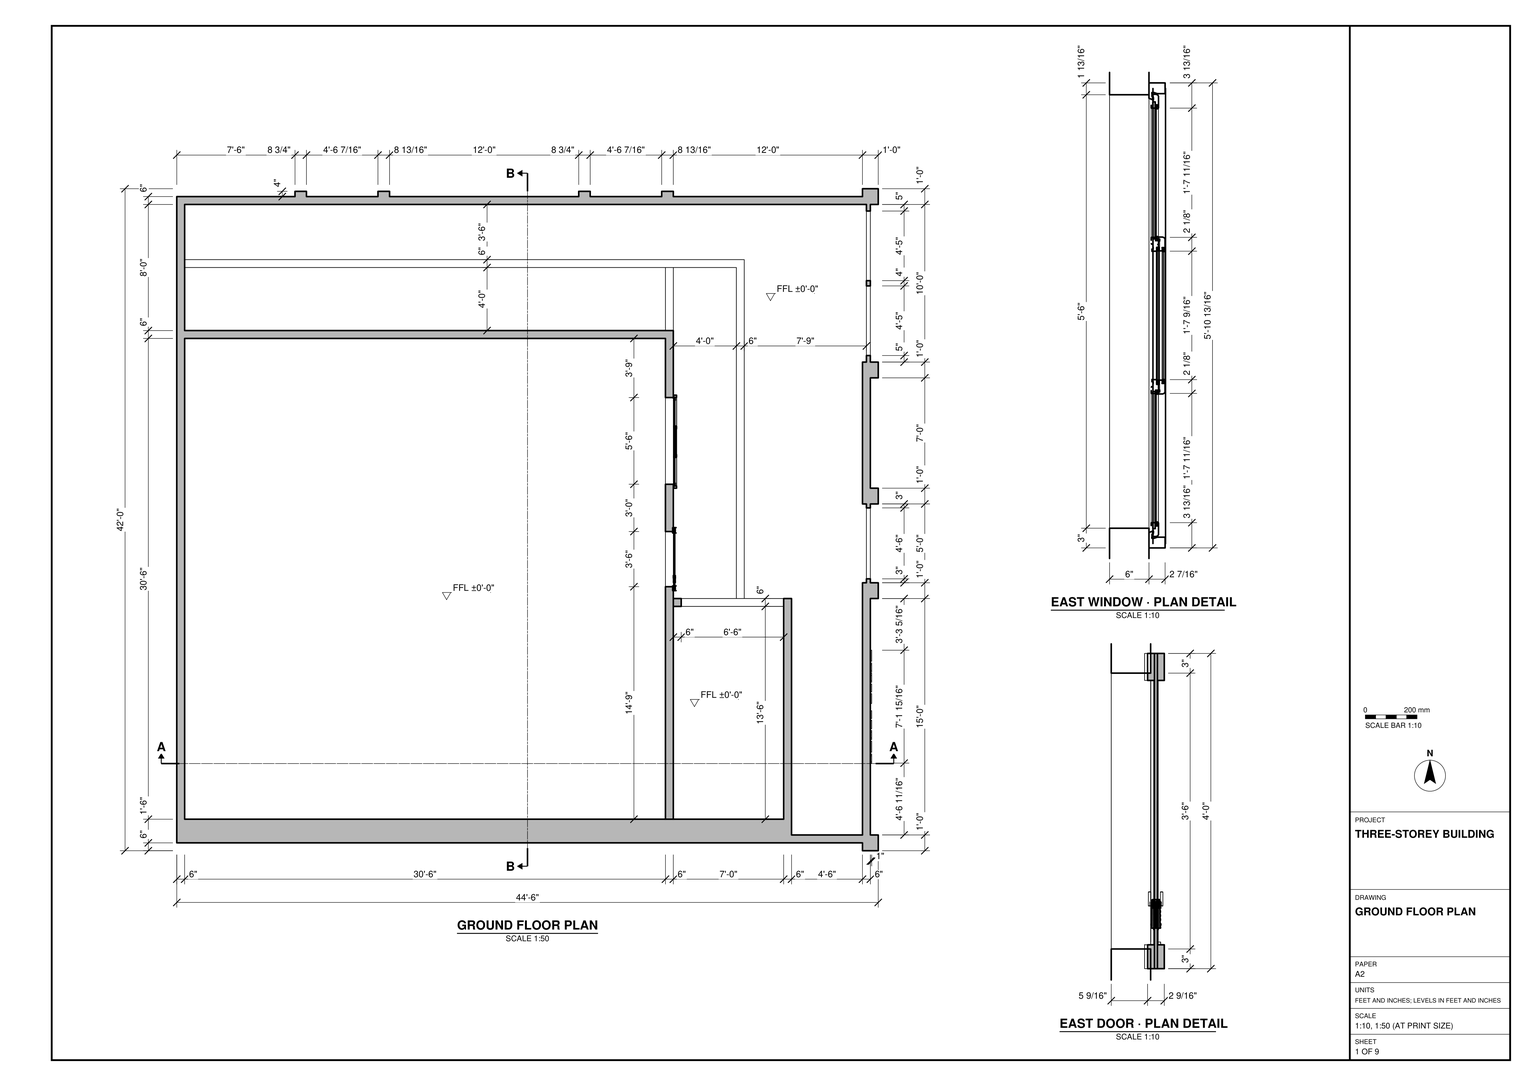
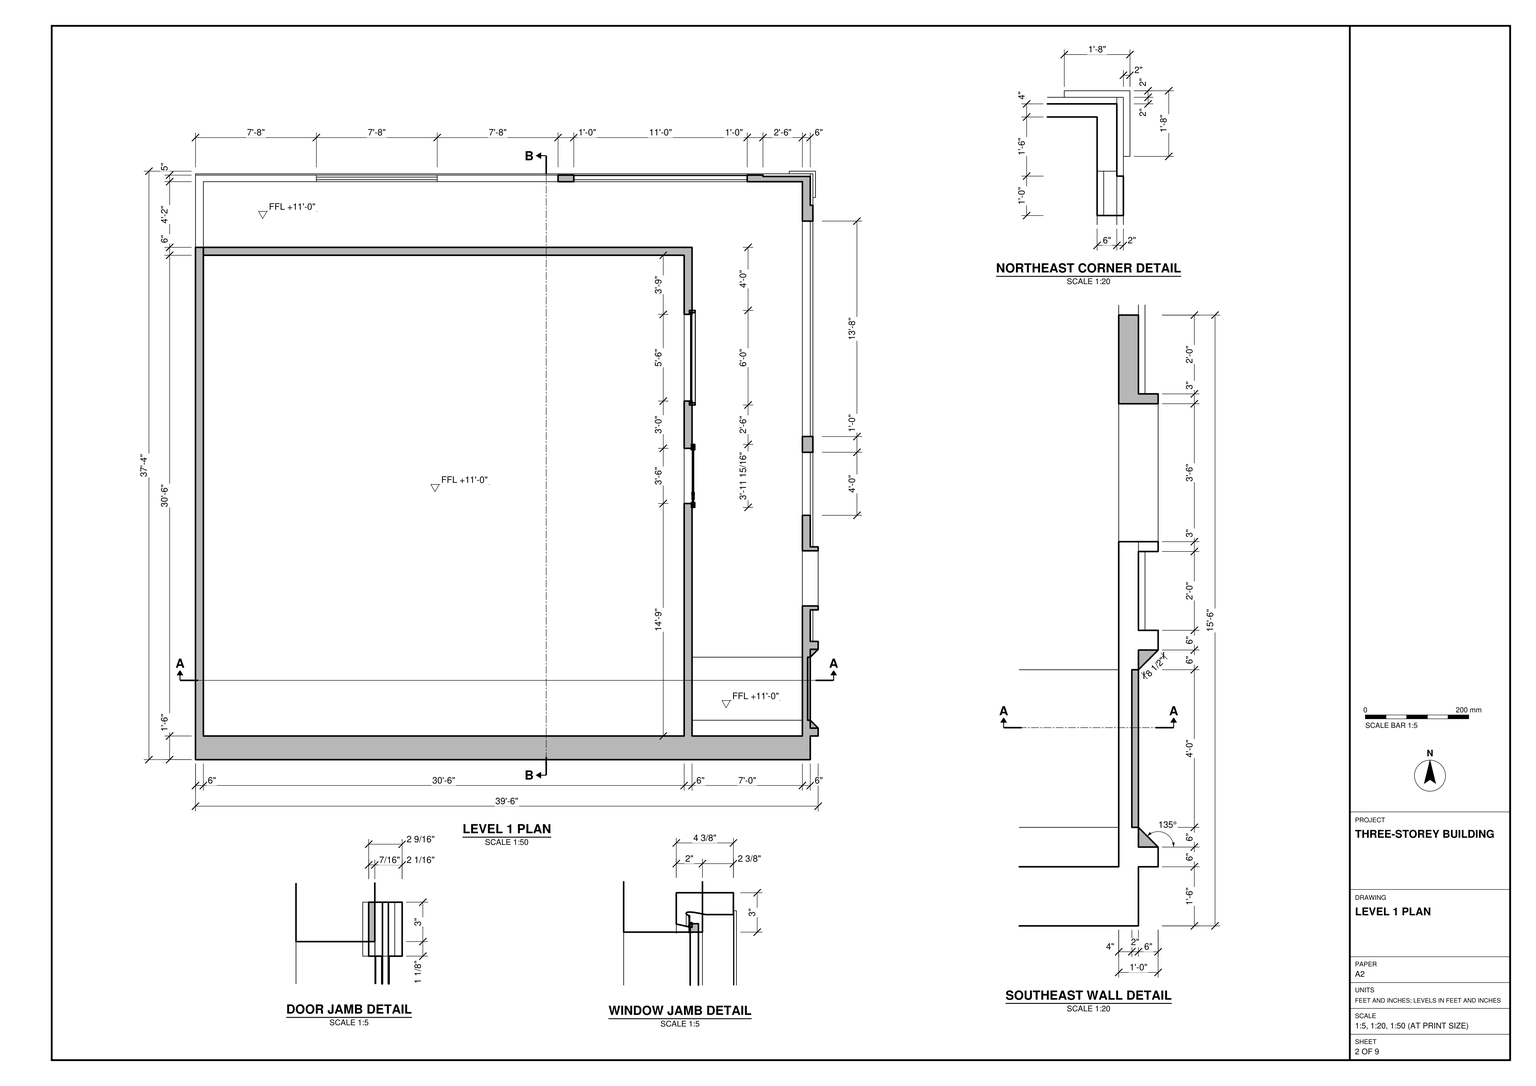
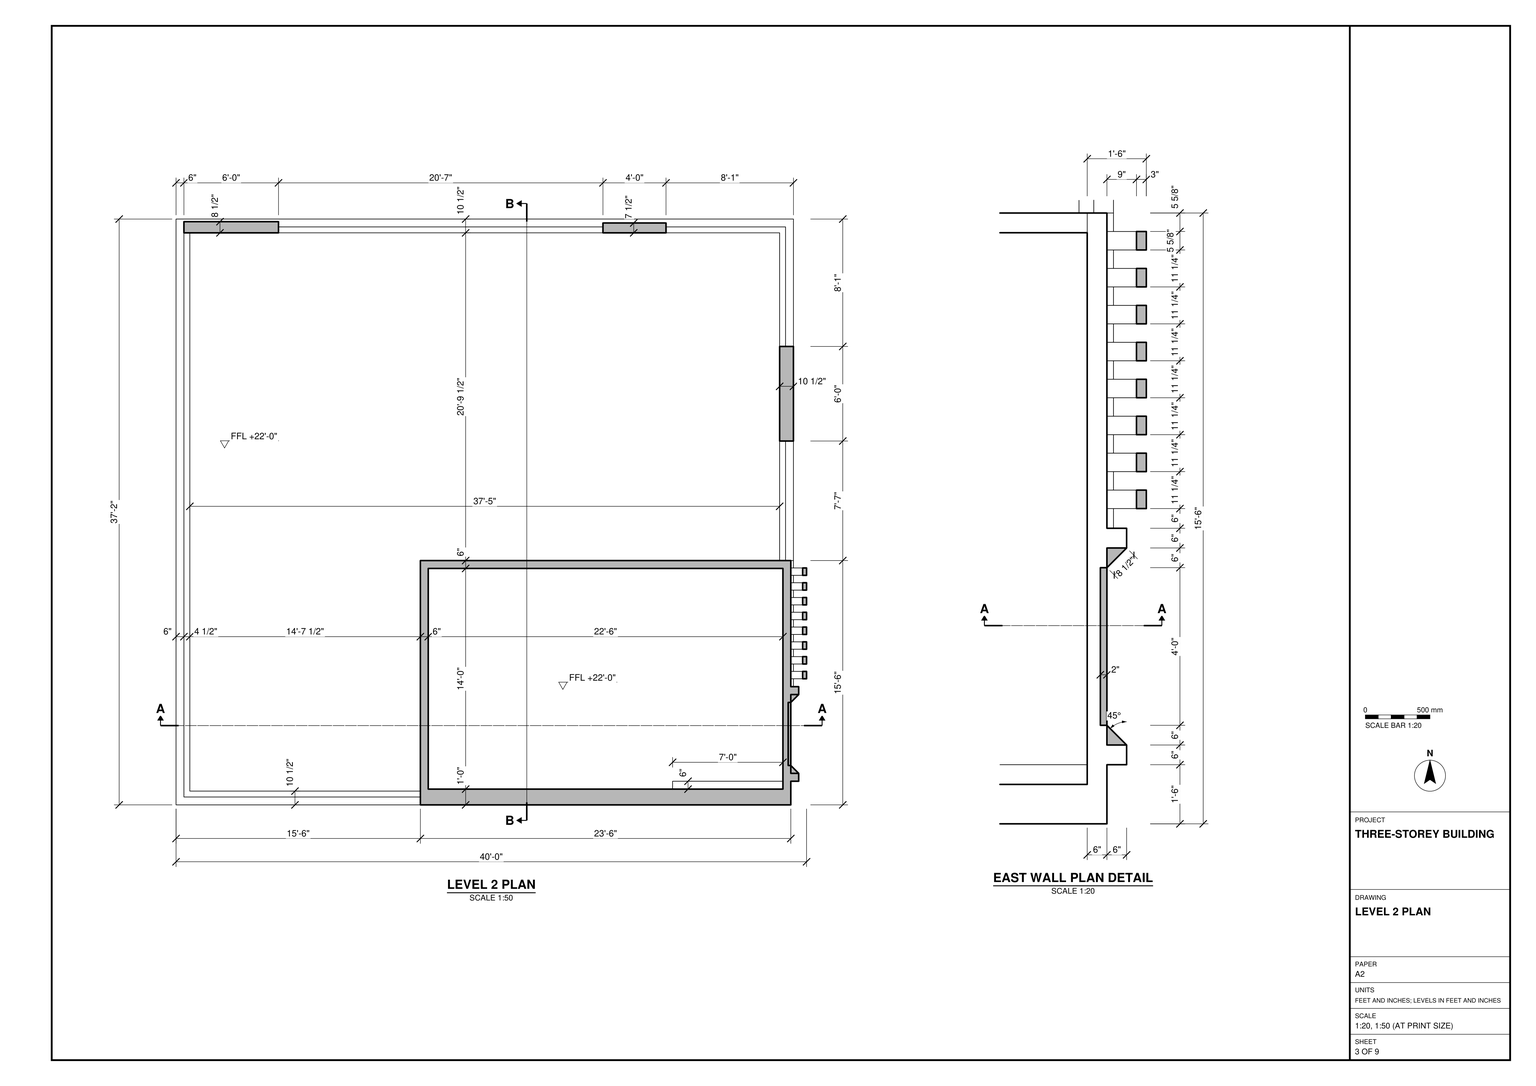
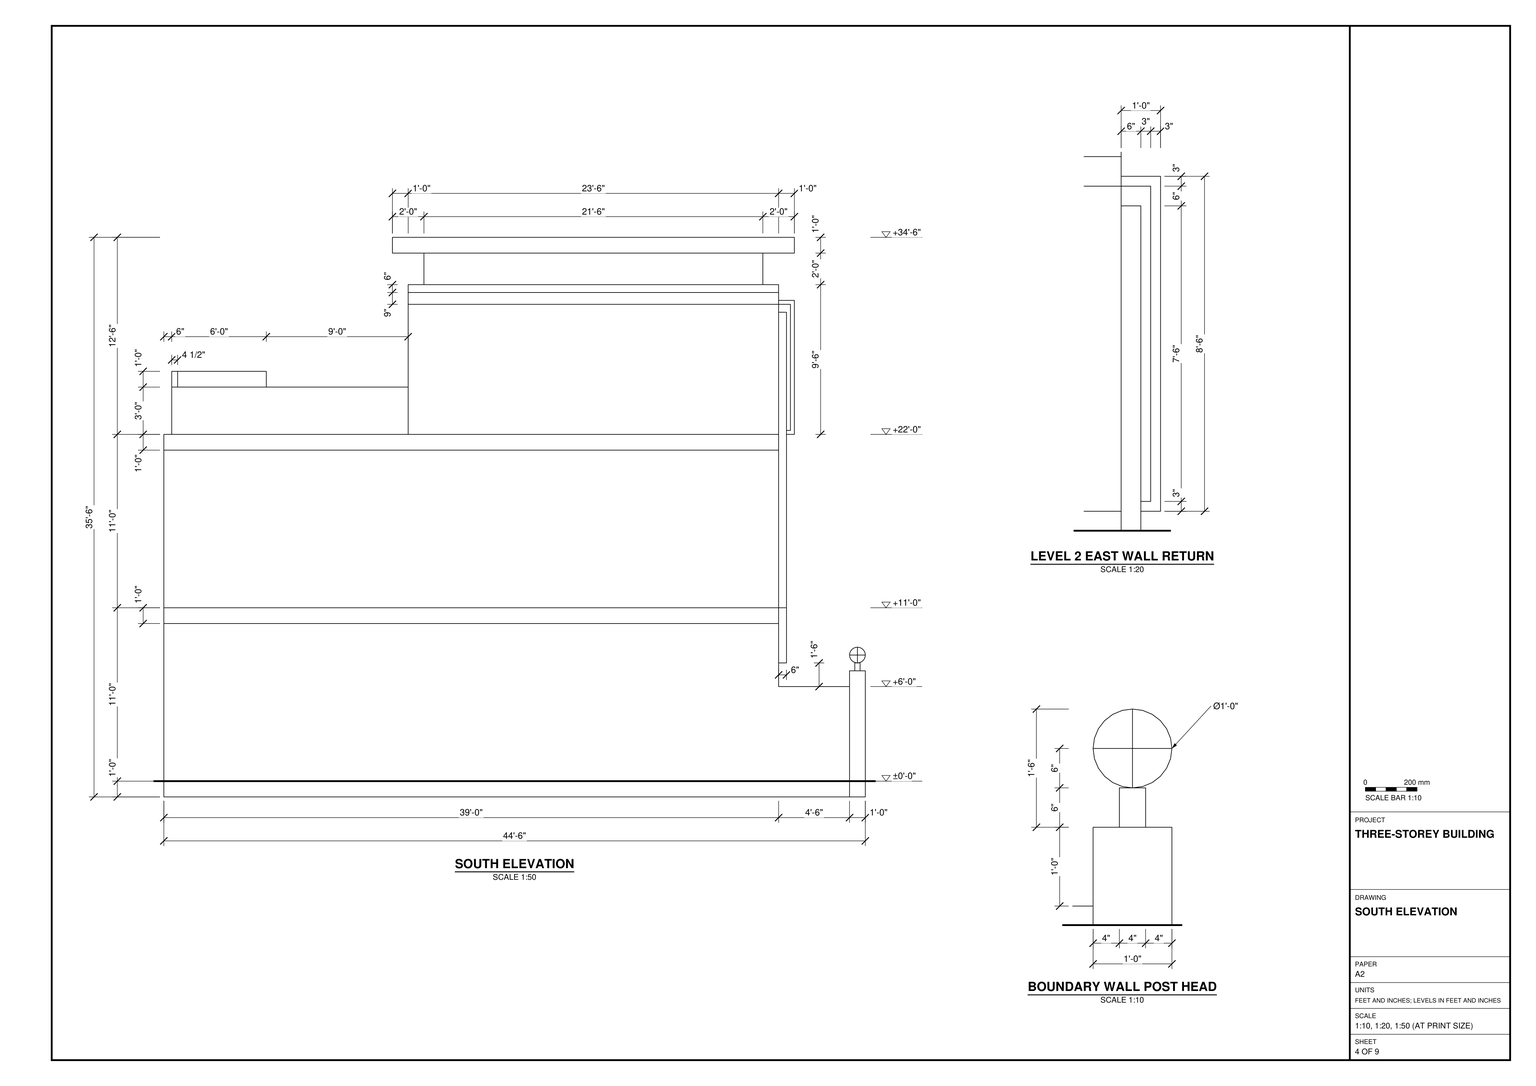
Build the three-storey building in SketchUp from task_files/diagram_01.pdf. Work in feet and inches. The overall dimensions, including projections, are 44'-6" east–west by 42'-6" north–south by 35'-6" high. Set the finished floors at ±0'-0", +11'-0" and +22'-0".

On the ground floor and Level 1, lay out the large square room with the narrower floor areas along its north and east sides. Follow the wall thicknesses shown in plan, including the thicker south wall. Use the ground-floor plan for the small southeast enclosure and the projecting perimeter piers. Fit the east-facing window and door units into the main room walls using the plan and jamb details.

Model the floor slabs to their respective outlines rather than copying the ground-floor perimeter upwards. On Level 2, place the roofed enclosure at the southeast corner, with the terrace extending north and west of it. Follow the east wall detail for the projecting fins and the recess with angled ends. Include stairs, built-in joinery and main furniture only where shown. Any decor or loose items shown may be suitable library components.

Keep walls, slabs, roof elements and each furniture or joinery piece in separate groups or components, and use components for repeated parts. Save one SketchUp model as output_files/stepped_three_storey_building_and_its_upper_terrace.skp.

# SketchUp Ruby script. Lengths in inches.
U = 1.inch
M = Sketchup.active_model
def pt(a) = Geom::Point3d.new(a.map { |v| v * U })
def face(e, loops, mat)
  f = e.add_face(loops[0].map { |a| pt(a) })
  loops[1..].each { |l| e.add_face(l.map { |a| pt(a) }).erase! }
  f.material = f.back_material = mat if mat
  f
end
# faces: each face lists its corners as indices into pts; further lists are holes
def faces(e, pts, list, mat = nil) = list.each { |f| face(e, (f[0].is_a?(Array) ? f : [f]).map { |l| l.map { |i| pts[i] } }, mat) }
# xy, xz, yz: faces in a plane at the given z, y or x. An outline is a flat list of corners, or four numbers for a rectangle; further outlines are holes
def ring(l) = l.size == 4 ? [[l[0], l[1]], [l[2], l[1]], [l[2], l[3]], [l[0], l[3]]] : l.each_slice(2).to_a
def flat(e, list, mat, &to3) = list.each { |f| face(e, (f[0].is_a?(Array) ? f : [f]).map { |l| ring(l).map { |u, v| to3.(u, v) } }, mat) }
def xy(e, z, list, mat = nil) = flat(e, list, mat) { |x, y| [x, y, z] }
def xz(e, y, list, mat = nil) = flat(e, list, mat) { |x, z| [x, y, z] }
def yz(e, x, list, mat = nil) = flat(e, list, mat) { |y, z| [x, y, z] }
def lines(e, pts, list) = list.each { |a, b| e.add_line(pt(pts[a]), pt(pts[b])) }
# prism: a flat outline (further loops are holes) pulled along v
def prism(e, loops, v, mat = nil)
  f = face(e, loops, mat); d = Geom::Vector3d.new(v.map { |x| x * U })
  f.pushpull(f.normal.samedirection?(d) ? d.length : -d.length)
end
def box(e, o, s, mat = nil) = prism(e, [[o, [o[0] + s[0], o[1], o[2]], [o[0] + s[0], o[1] + s[1], o[2]], [o[0], o[1] + s[1], o[2]]]], [0, 0, s[2]], mat)
def at(x, y, z, deg = 0) = Geom::Transformation.translation(pt([x, y, z])) * Geom::Transformation.rotation(ORIGIN, Z_AXIS, deg.degrees)
def axes(o, x, y, z) = Geom::Transformation.new([*x, 0, *y, 0, *z, 0, *pt(o).to_a, 1])
def part(name) = M.definitions.add(name)
# library, detail: a bought-in or finely detailed component or shape, given as its bounding box
def library(name, o, s) = part(name).tap { |d| box(d.entities, o, s) }
def detail(e, o, s) = box(e.add_group.entities, o, s)
def put(e, d, t, mat = nil) = e.add_instance(d, t).tap { |i| i.material = mat if mat }
def group(e, t, mat = nil) = e.add_group.tap { |g| g.transformation = t; g.material = mat if mat }.entities
root = M.entities
M.materials.add("Brick_20_1K").color = [126, 119, 119]
M.materials.add("D01_Frost_White").color = [255, 255, 255]
M.materials.add("D02_Buttercup_Glow").color = [255, 229, 155]
M.materials.add("Glass_Basic_01").color = [186, 168, 28]
M.materials["Glass_Basic_01"].alpha = 0.25
M.materials.add("Glass_Basic_1").color = [161, 173, 186]
M.materials["Glass_Basic_1"].alpha = 0.25
M.materials.add("M08_Obsidian_Black").color = [30, 30, 30]
M.materials.add("M09_Shadow_Night").color = [0, 0, 0]
M.materials.add("ThomThom - Buttons2").color = [40, 40, 43]
M.materials.add("ThomThom - Hat2").color = [38, 38, 38]
M.materials.add("ThomThom - Waistcoat2").color = [127, 127, 126]
c1 = library("mesh-164",[-1582.71,-3144.16,-23.22],[2366.42,2227.34,65.81])
c2 = part("Group13")
put(c2.entities,c1,at(294.66,859.51,3.5))
c3 = library("HOUSE DEKHO",[0.96,0,0],[85.97,9.9,1])
c4 = library("Sphere Light",[-6,-6,-6],[12,12,12])
c5 = library("Sphere Light\#1",[-6,-6,-6],[12,12,12])
c6 = library("Sphere Light\#2",[-6,-6,-6],[12,12,12])
c7 = library("Sphere Light\#3",[-6,-6,-6],[12,12,12])
c8 = library("porta+4",[0.2,-5.42,1.33],[46.55,4.72,83.21])
put(root,c2,axes([378.78,320.54,109.87],[0,0.02992,0],[0,0,0.03268],[0.03937,0,0]))
put(root,c2,axes([377.38,321.19,235.38],[0,0.03043,0],[0,0,0.02406],[0.06969,0,0]))
g1 = group(root,at(0,24,0),"D01_Frost_White")
xy(g1,0,[[522,-18,522,-12,528,-12,528,-6,534,-6,534,-18],[0,-12,0,480,90,480,90,484,98.72,484,98.72,480,153.16,480,153.16,484,162,484,162,480,306,480,306,484,314.72,484,314.72,480,369.16,480,369.16,484,378,484,378,480,528,480,528,-12],[528,174,534,186],[528,246,534,258],[528,342,534,354],
  [528,474,528,480,522,480,522,486,534,486,534,474]])
xy(g1,3,[[525,189,528,243]],"M08_Obsidian_Black")
xy(g1,5,[[525,359,528,412],[525,416,528,469]],"M08_Obsidian_Black")
xy(g1,6.39,[[525,189,528,243]],"M08_Obsidian_Black")
xy(g1,8.22,[[525,359,528,412],[525,416,528,469]])
xy(g1,9.78,[[525,189,528,243]],"M08_Obsidian_Black")
xy(g1,11.43,[[525,359,528,412],[525,416,528,469]],"M08_Obsidian_Black")
xy(g1,12,[[468,-6,522,-6,522,186,525,186,525,246,522,246,522,354,525,354,525,474,6,474,6,432,432,432,432,174,468,174],[6,6,372,372],[378,6,462,168],[426,174,432,174,432,432,6,432,6,426,426,426],[378,174,426,426],
  [6,378,372,426],[372,378,378,426]])
xy(g1,13.17,[[525,189,528,243]],"M08_Obsidian_Black")
xy(g1,14.65,[[525,359,528,412],[525,416,528,469]])
xy(g1,15,[[372,183,378,225]])
xy(g1,16.57,[[525,189,528,243]],"M08_Obsidian_Black")
xy(g1,17.87,[[525,359,528,412],[525,416,528,469]],"M08_Obsidian_Black")
xy(g1,18,[[384,168,462,174]])
xy(g1,19.96,[[525,189,528,243]],"M08_Obsidian_Black")
xy(g1,21.09,[[525,359,528,412],[525,416,528,469]])
xy(g1,23.35,[[525,189,528,243]],"M08_Obsidian_Black")
xy(g1,24.3,[[525,359,528,412],[525,416,528,469]],"M08_Obsidian_Black")
xy(g1,26.74,[[525,189,528,243]],"M08_Obsidian_Black")
xy(g1,27.52,[[525,359,528,412],[525,416,528,469]])
xy(g1,30.13,[[525,189,528,243]],"M08_Obsidian_Black")
xy(g1,30.74,[[525,359,528,412],[525,416,528,469]],"M08_Obsidian_Black")
xy(g1,33.52,[[525,189,528,243]],"M08_Obsidian_Black")
xy(g1,33.96,[[525,359,528,412],[525,416,528,469]])
xy(g1,36.91,[[525,189,528,243]],"M08_Obsidian_Black")
xy(g1,37.17,[[525,359,528,412],[525,416,528,469]],"M08_Obsidian_Black")
xy(g1,40.3,[[525,189,528,243]],"M08_Obsidian_Black")
xy(g1,40.39,[[525,359,528,412],[525,416,528,469]])
xy(g1,43.61,[[525,359,528,412],[525,416,528,469]],"M08_Obsidian_Black")
xy(g1,43.7,[[525,189,528,243]],"M08_Obsidian_Black")
xy(g1,46.83,[[525,359,528,412],[525,416,528,469]])
xy(g1,47.09,[[525,189,528,243]],"M08_Obsidian_Black")
xy(g1,50.04,[[525,359,528,412],[525,416,528,469]],"M08_Obsidian_Black")
xy(g1,50.48,[[525,189,528,243]],"M08_Obsidian_Black")
xy(g1,53.26,[[525,359,528,412],[525,416,528,469]])
xy(g1,53.87,[[525,189,528,243]],"M08_Obsidian_Black")
xy(g1,56.48,[[525,359,528,412],[525,416,528,469]],"M08_Obsidian_Black")
xy(g1,57,[[372,261,378,327]])
xy(g1,57.26,[[525,189,528,243]],"M08_Obsidian_Black")
xy(g1,59.7,[[525,359,528,412],[525,416,528,469]])
xy(g1,60.65,[[525,189,528,243]],"M08_Obsidian_Black")
xy(g1,62.91,[[525,359,528,412],[525,416,528,469]],"M08_Obsidian_Black")
xy(g1,64.04,[[525,189,528,243]],"M08_Obsidian_Black")
xy(g1,66.13,[[525,359,528,412],[525,416,528,469]])
xy(g1,67.43,[[525,189,528,243]],"M08_Obsidian_Black")
xy(g1,69.35,[[525,359,528,412],[525,416,528,469]],"M08_Obsidian_Black")
xy(g1,70.83,[[525,189,528,243]],"M08_Obsidian_Black")
xy(g1,72.57,[[525,359,528,412],[525,416,528,469]])
xy(g1,74.22,[[525,189,528,243]],"M08_Obsidian_Black")
xy(g1,75.78,[[525,359,528,412],[525,416,528,469]],"M08_Obsidian_Black")
xy(g1,77.61,[[525,189,528,243]],"M08_Obsidian_Black")
xy(g1,79,[[525,359,528,412],[525,416,528,469]])
xy(g1,81,[[525,189,528,243]],"M08_Obsidian_Black")
xy(g1,82,[[0,480,90,482],[162,480,306,482],[378,480,522,482]],"M08_Obsidian_Black")
xy(g1,82,[[528,258,530,342]],"ThomThom - Hat2")
xy(g1,84,[[468,-12,522,-6],[522,-6,528,174],[522,258,530,342],[0,378,6,378,6,474,90,474,90,482,0,482],[162,474,306,482],
  [378,474,522,482]])
xy(g1,84,[[525,186,528,246],[525,354,528,474]],"M08_Obsidian_Black")
xy(g1,89.61,[[98.72,480,153.16,484],[314.72,480,369.16,484]])
xy(g1,96,[[522,-18,534,-6],[[522,174,534,186],[526,178,530,182]],[[522,246,534,258],[526,250,530,254]],[[522,342,534,354],[526,346,530,350]],[90,474,162,484],
  [306,474,378,484],[[522,474,534,486],[526,478,530,482]]])
xy(g1,102,[[468,6,474,78],[526,178,528,180],[528,178,530,180],[526,180,528,182],[528,180,530,182],
  [526,250,530,254],[526,346,530,350],[526,478,530,482]])
xy(g1,105,[[372,183,378,225],[372,261,378,327]])
xy(g1,108,[[468,12,474,72]])
xy(g1,114,[[466,18,468,66]],"D02_Buttercup_Glow")
xy(g1,120,[[464,174,464,428,0,428,0,434,470,434,470,174]])
xy(g1,126,[[384,168,462,174]])
xy(g1,126.05,[[470,416,470,434,452,434,452,436,472,436,472,416]])
xy(g1,127.54,[[470,416,472,416,472,436,452,436,452,434,470,434]])
xy(g1,129.03,[[470,416,470,434,452,434,452,436,472,436,472,416]])
xy(g1,130.52,[[470,416,472,416,472,436,452,436,452,434,470,434]])
xy(g1,132,[[0,-12,6,378],[6,6,372,372],[372,6,378,372],[378,6,462,168],[468,78,470,168],
  [378,168,468,174],[468,168,470,174],[378,174,378,378,6,378,6,428,12,428,12,384,384,384,384,180,464,180,464,174],[384,180,384,384,12,384,12,428,464,428,464,180],[6,372,378,378],
  [0,378,6,428]])
xy(g1,135,[[468,78,470,434],[0,432,468,434]])
xy(g1,141,[[468,78,470,174],[468,174,468,432,0,432,0,434,470,434,470,174]])
xy(g1,144,[[6,6,372,372],[378,6,462,18],[378,18,462,66],[378,66,462,66,462,428,6,428,6,378,378,378],[468,78,470,222],
  [468,410,470,434],[432,432,468,432,468,434,0,434,0,433,432,433]])
xy(g1,147,[[372,183,378,225]])
xy(g1,150,[[92,428,184,433]])
xy(g1,154.2,[[92,429.5,184,431.5]])
xy(g1,156,[[468,234,470,398],[288,428,420,429.5],[288,432.5,420,433]])
xy(g1,156.9,[[92,429.5,184,431.5]])
xy(g1,157,[[462,235,468,397],[289,429.5,419,432.5]])
xy(g1,159.6,[[92,429.5,184,431.5]])
xy(g1,162.3,[[92,429.5,184,431.5]])
xy(g1,165,[[92,429.5,184,431.5]])
xy(g1,167.7,[[92,429.5,184,431.5]])
xy(g1,170.4,[[92,429.5,184,431.5]])
xy(g1,173.1,[[92,429.5,184,431.5]])
xy(g1,175.8,[[92,429.5,184,431.5]])
xy(g1,178.5,[[92,429.5,184,431.5]])
xy(g1,179,[[462,235,468,397],[289,429.5,419,432.5]])
xy(g1,180,[[468,102,474,150],[462,174,468,222],[462,222,468,234],[462,234,468,398],[0,378,6,378,6,428,92,428,92,433,0,433],
  [184,428,276,433],[288,429.5,420,432.5]])
xy(g1,181.5,[[462,411.5,468,411.5,468,432,433.5,432,433.5,428,462,428]])
xy(g1,182.74,[[462,411.5,462,428,433.5,428,433.5,432,468,432,468,411.5]])
xy(g1,183,[[462,105,474,147],[372,261,378,327]])
xy(g1,189.97,[[462,411.5,468,411.5,468,432,433.5,432,433.5,428,462,428]])
xy(g1,191.21,[[462,411.5,462,428,433.5,428,433.5,432,468,432,468,411.5]])
xy(g1,198.44,[[462,411.5,468,411.5,468,432,433.5,432,433.5,428,462,428]])
xy(g1,199.68,[[462,411.5,462,428,433.5,428,433.5,432,468,432,468,411.5]])
xy(g1,206.91,[[462,411.5,468,411.5,468,432,433.5,432,433.5,428,462,428]])
xy(g1,208.15,[[462,411.5,462,428,433.5,428,433.5,432,468,432,468,411.5]])
xy(g1,215.38,[[462,411.5,468,411.5,468,432,433.5,432,433.5,428,462,428]])
xy(g1,216.62,[[462,411.5,462,428,433.5,428,433.5,432,468,432,468,411.5]])
xy(g1,223.85,[[462,411.5,468,411.5,468,432,433.5,432,433.5,428,462,428]])
xy(g1,225.09,[[462,411.5,462,428,433.5,428,433.5,432,468,432,468,411.5]])
xy(g1,231,[[372,261,378,327]])
xy(g1,232.32,[[462,411.5,468,411.5,468,432,433.5,432,433.5,428,462,428]])
xy(g1,233.56,[[462,411.5,462,428,433.5,428,433.5,432,468,432,468,411.5]])
xy(g1,237,[[462,105,474,147],[372,183,378,225]])
xy(g1,240,[[468,102,474,150]])
xy(g1,240.79,[[462,411.5,468,411.5,468,432,433.5,432,433.5,428,462,428]])
xy(g1,242.03,[[462,411.5,462,428,433.5,428,433.5,432,468,432,468,411.5]])
xy(g1,249.26,[[462,411.5,468,411.5,468,432,433.5,432,433.5,428,462,428]])
xy(g1,250.5,[[462,411.5,462,428,433.5,428,433.5,432,468,432,468,411.5]])
xy(g1,252,[[462,234,470,398],[288,428,420,433]])
xy(g1,264,[[0,-12,6,378],[6,6,372,372],[372,6,378,174],[378,6,462,18],[378,18,462,66],
  [378,66,378,378,6,378,6,434,276,434,276,428,462,428,462,222,470,222,470,174,462,174,462,66],[468,78,470,84],[468,84,470,174],[372,174,378,174,378,378,6,378,6,372,372,372],[462,222,470,410],
  [0,378,6,434],[462,410,468,410,468,432,432,432,432,433,276,433,276,428,462,428],[468,410,468,432,432,432,432,434,470,434,470,410],[276,433,432,434]])
xy(g1,267,[[468,78,470,78,470,434,0,434,0,432,468,432]])
xy(g1,273,[[468,78,470,89.625],[468,89.625,470,95.25],[468,95.25,470,100.875],[468,100.875,470,106.5],[468,106.5,470,112.125],
  [468,112.125,470,117.75],[468,117.75,470,123.375],[468,123.375,470,129],[468,129,470,134.625],[468,134.625,470,140.25],
  [468,140.25,470,145.875],[468,145.875,470,151.5],[468,151.5,470,157.125],[468,157.125,470,162.75],[468,162.75,470,168.375],
  [468,168.375,470,174],[468,174,470,434],[0,432,468,434]])
xy(g1,276,[[0,-12,186,-12,186,-6,6,-6,6,432,10.5,432,10.5,428,73.5,428,73.5,432,78,432,78,428,325,428,325,431,329.5,431,329.5,428,368.5,428,368.5,431,373,431,373,428,464,428,464,337,470,337,470,434,0,434],[186,-12,378,-12,378,0,192,0,192,168,186,168],[10.5,-1.5,186,-1.5,186,174,459.5,174,459.5,423.5,10.5,423.5],[192,0,378,0,378,6,462,6,462,168,192,168],[378,0,462,6],
  [468,78,470,84],[470,84,480,89.625],[468,89.625,470,95.25],[470,95.25,480,100.875],[468,100.875,470,106.5],
  [470,106.5,480,112.125],[468,112.125,470,117.75],[470,117.75,480,123.375],[468,123.375,470,129],[470,129,480,134.625],
  [468,134.625,470,140.25],[470,140.25,480,145.875],[468,145.875,470,151.5],[470,151.5,480,157.125],[468,157.125,470,162.75],
  [470,162.75,480,168.375],[186,168,462,174],[468,168.375,470,174],[464,174,470,265],[464,269.5,470,332.5]])
xy(g1,279,[[468,84,477,89.625],[468,95.25,477,100.875],[468,106.5,477,112.125],[468,117.75,477,123.375],[468,129,477,134.625],
  [468,140.25,477,145.875],[468,151.5,477,157.125],[468,162.75,477,168.375]])
xy(g1,291,[[459.5,174,464,222],[459.5,392,464,392,464,428,416,428,416,423.5,459.5,423.5],[182.67,423.5,254.67,428]])
xy(g1,297,[[459.5,174,464,222],[459.5,392,464,428],[182.67,423.5,254.67,428],[416,423.5,459.5,428]])
xy(g1,312,[[6,-6,186,-6,186,-1.5,10.5,-1.5,10.5,423.5,6,423.5],[459.5,174,464,265],[459.5,337,464,337,464,428,373,428,373,423.5,459.5,423.5],[78,423.5,325,428]])
xy(g1,319.5,[[464,269.5,470,332.5],[10.5,428,73.5,432],[329.5,428,368.5,431]])
xy(g1,324,[[459.5,265,470,269.5],[459.5,269.5,470,337],[6,423.5,78,432],[325,423.5,373,431]])
xy(g1,357,[[466,18,468,66]],"D02_Buttercup_Glow")
xy(g1,363,[[468,12,474,72]])
xy(g1,369,[[468,6,474,78]])
xy(g1,375,[[468,84,477,89.625],[468,95.25,477,100.875],[468,106.5,477,112.125],[468,117.75,477,123.375],[468,129,477,134.625],
  [468,140.25,477,145.875],[468,151.5,477,157.125],[468,162.75,477,168.375]])
xy(g1,378,[[468,84,480,89.625],[468,95.25,480,100.875],[468,106.5,480,112.125],[468,117.75,480,123.375],[468,129,480,134.625],
  [468,140.25,480,145.875],[468,151.5,480,157.125],[468,162.75,480,168.375]])
xy(g1,384,[[186,-12,468,0],[186,0,192,174],[192,0,462,168],[462,0,468,174],[192,168,462,174]])
xy(g1,390,[[[186,-12,468,174],[198,0,456,162]],[204,6,450,156]])
xy(g1,414,[[174,-24,198,6],[[198,-24,198,0,456,0,456,162,198,162,198,6,174,6,174,234,480,234,480,-24],[186,174,226.29,222],[347.14,174,387.43,222],[427.71,174,468,222],[266.57,174,306.86,222]],[198,0,450,6],[450,0,456,162],[198,6,204,162],
  [204,6,450,156],[204,156,450,162]])
xy(g1,426,[[[174,-24,480,234],[427.71,174,468,222],[347.14,174,387.43,222],[266.57,174,306.86,222],[186,174,226.29,222]]])
xz(g1,-24,[[174,414,480,426]])
xz(g1,-18,[[522,0,534,96]])
xz(g1,-12,[[0,0,522,0,522,84,468,84,468,132,0,132],[0,144,468,264],[186,276,468,375],[186,375,468,384]])
xz(g1,-12,[[186,384,468,390]],"M08_Obsidian_Black")
xz(g1,-12,[[0,132,468,144],[0,264,468,276]],"ThomThom - Hat2")
xz(g1,-6,[[528,0,534,96],[468,12,522,84],[522,84,528,96],[6,276,186,312]])
xz(g1,-1.5,[[10.5,276,186,312]])
xz(g1,0,[[192,276,462,384],[198,390,456,414]])
xz(g1,6,[[6,12,372,132],[372,12,378,132],[378,12,462,132],[468,102,474,144],[6,144,372,264],
  [378,144,462,264],[468,144,474,369],[378,264,462,276],[204,390,450,414]])
xz(g1,12,[[468,108,474,363]])
xz(g1,18,[[466,114,468,357]],"D02_Buttercup_Glow")
xz(g1,66,[[466,114,468,357]],"D02_Buttercup_Glow")
xz(g1,72,[[468,108,474,264],[468,264,474,276],[468,276,474,363]])
xz(g1,78,[[468,102,468,132,470,132,470,135,468,135,468,141,470,141,470,144,468,144,468,264,474,264,474,102],[470,264,470,267,468,267,468,273,470,273,470,276,474,276,474,264],[468,276,474,369]])
xz(g1,84,[[468,276,480,276,480,378,468,378,468,375,477,375,477,279,468,279]])
xz(g1,89.625,[[468,276,468,279,477,279,477,375,468,375,468,378,480,378,480,276]])
xz(g1,95.25,[[468,276,480,276,480,378,468,378,468,375,477,375,477,279,468,279]])
xz(g1,100.875,[[468,276,468,279,477,279,477,375,468,375,468,378,480,378,480,276]])
xz(g1,102,[[468,180,474,240]])
xz(g1,105,[[462,183,474,237]])
xz(g1,106.5,[[468,276,480,276,480,378,468,378,468,375,477,375,477,279,468,279]])
xz(g1,112.125,[[468,276,468,279,477,279,477,375,468,375,468,378,480,378,480,276]])
xz(g1,117.75,[[468,276,480,276,480,378,468,378,468,375,477,375,477,279,468,279]])
xz(g1,123.375,[[468,276,468,279,477,279,477,375,468,375,468,378,480,378,480,276]])
xz(g1,129,[[468,276,480,276,480,378,468,378,468,375,477,375,477,279,468,279]])
xz(g1,134.625,[[468,276,468,279,477,279,477,375,468,375,468,378,480,378,480,276]])
xz(g1,140.25,[[468,276,480,276,480,378,468,378,468,375,477,375,477,279,468,279]])
xz(g1,145.875,[[468,276,468,279,477,279,477,375,468,375,468,378,480,378,480,276]])
xz(g1,147,[[462,183,474,237]])
xz(g1,150,[[468,180,474,240]])
xz(g1,151.5,[[468,276,480,276,480,378,468,378,468,375,477,375,477,279,468,279]])
xz(g1,156,[[204,390,450,414]])
xz(g1,157.125,[[468,276,468,279,477,279,477,375,468,375,468,378,480,378,480,276]])
xz(g1,162,[[198,390,456,414]])
xz(g1,162.75,[[468,276,480,276,480,378,468,378,468,375,477,375,477,279,468,279]])
xz(g1,168,[[378,12,462,12,462,18,384,18,384,126,462,126,462,132,378,132],[192,276,462,384]])
xz(g1,168.375,[[468,276,468,279,477,279,477,375,468,375,468,378,480,378,480,276]])
xz(g1,174,[[528,0,534,0,534,96,522,96,522,84,528,84],[[378,12,378,132,464,132,464,120,468,120,468,12],[384,18,462,126]],[464,120,468,132],[468,120,470,132],[462,180,468,264],
  [459.5,276,462,291],[459.5,297,462,312],[186,414,204,426],[204,414,226.29,426],[266.57,414,306.86,426],
  [347.14,414,387.43,426],[427.71,414,450,426],[450,414,456,426],[456,414,468,426]])
xz(g1,174,[[[186,276,186,384,468,384,468,276,464,276,464,291,459.5,291,459.5,276],[459.5,297,464,312]],[186,384,468,390]],"M08_Obsidian_Black")
xz(g1,178,[[526,96,530,102]])
xz(g1,182,[[526,96,530,102]])
xz(g1,183,[[372,15,378,105],[372,147,378,237]])
xz(g1,186,[[528,0,528,84,522,84,522,96,534,96,534,0],[522,12,525,84]])
xz(g1,189,[[525,3,528,6.39],[525,9.78,528,13.17],[525,16.57,528,19.96],[525,23.35,528,26.74],[525,30.13,528,33.52],
  [525,36.91,528,40.3],[525,43.7,528,47.09],[525,50.48,528,53.87],[525,57.26,528,60.65],[525,64.04,528,67.43],
  [525,70.83,528,74.22],[525,77.61,528,81]])
xz(g1,222,[[468,144,470,264],[462,180,468,264],[459.5,291,464,297],[186,414,226.29,426],[266.57,414,306.86,426],
  [347.14,414,387.43,426],[427.71,414,468,426]])
xz(g1,225,[[372,15,378,105],[372,147,378,237]])
xz(g1,234,[[462,156,468,180],[468,156,468,180,462,180,462,252,470,252,470,156],[174,414,480,426]])
xz(g1,235,[[462,157,468,179]])
xz(g1,243,[[525,3,528,6.39],[525,9.78,528,13.17],[525,16.57,528,19.96],[525,23.35,528,26.74],[525,30.13,528,33.52],
  [525,36.91,528,40.3],[525,43.7,528,47.09],[525,50.48,528,53.87],[525,57.26,528,60.65],[525,64.04,528,67.43],
  [525,70.83,528,74.22],[525,77.61,528,81]])
xz(g1,246,[[528,0,534,0,534,96,522,96,522,84,528,84],[522,12,525,84]])
xz(g1,250,[[526,96,530,102]])
xz(g1,254,[[526,96,530,102]])
xz(g1,258,[[528,0,528,82,530,82,530,84,522,84,522,96,534,96,534,0]])
xz(g1,261,[[372,57,378,105],[372,183,378,231]])
xz(g1,265,[[464,276,470,276,470,324,459.5,324,459.5,312,464,312]])
xz(g1,269.5,[[464,276,470,319.5]])
xz(g1,327,[[372,57,378,105],[372,183,378,231]])
xz(g1,332.5,[[464,276,470,319.5]])
xz(g1,337,[[464,276,464,312,459.5,312,459.5,324,470,324,470,276]])
xz(g1,342,[[528,0,534,0,534,96,522,96,522,84,530,84,530,82,528,82]])
xz(g1,346,[[526,96,530,102]])
xz(g1,350,[[526,96,530,102]])
xz(g1,354,[[528,0,528,84,525,84,525,12,522,12,522,96,534,96,534,0]])
xz(g1,359,[[525,5,528,8.22],[525,11.43,528,14.65],[525,17.87,528,21.09],[525,24.3,528,27.52],[525,30.74,528,33.96],
  [525,37.17,528,40.39],[525,43.61,528,46.83],[525,50.04,528,53.26],[525,56.48,528,59.7],[525,62.91,528,66.13],
  [525,69.35,528,72.57],[525,75.78,528,79]],"M08_Obsidian_Black")
xz(g1,372,[[6,12,372,132],[6,144,372,264]])
xz(g1,378,[[6,12,372,132],[372,12,378,132],[0,84,6,132],[6,144,378,264],[0,180,6,264]])
xz(g1,392,[[459.5,291,464,297]])
xz(g1,397,[[462,157,468,179]])
xz(g1,398,[[468,156,470,180],[462,180,470,252]])
xz(g1,410,[[468,144,470,180],[468,180,470,264]])
xz(g1,411.5,[[462,181.5,468,182.74],[462,189.97,468,191.21],[462,198.44,468,199.68],[462,206.91,468,208.15],[462,215.38,468,216.62],
  [462,223.85,468,225.09],[462,232.32,468,233.56],[462,240.79,468,242.03],[462,249.26,468,250.5]])
xz(g1,412,[[525,5,528,8.22]])
xz(g1,412,[[525,11.43,528,14.65],[525,17.87,528,21.09],[525,24.3,528,27.52],[525,30.74,528,33.96],[525,37.17,528,40.39],
  [525,43.61,528,46.83],[525,50.04,528,53.26],[525,56.48,528,59.7],[525,62.91,528,66.13],[525,69.35,528,72.57],
  [525,75.78,528,79]],"M08_Obsidian_Black")
xz(g1,416,[[470,126.05,472,127.54],[470,129.03,472,130.52]])
xz(g1,416,[[525,5,528,8.22],[525,11.43,528,14.65],[525,17.87,528,21.09],[525,24.3,528,27.52],[525,30.74,528,33.96],
  [525,37.17,528,40.39],[525,43.61,528,46.83],[525,50.04,528,53.26],[525,56.48,528,59.7],[525,62.91,528,66.13],
  [525,69.35,528,72.57],[525,75.78,528,79]],"M08_Obsidian_Black")
xz(g1,423.5,[[[10.5,276,459.5,276,459.5,291,416,291,416,297,459.5,297,459.5,312,373,312,373,324,325,324,325,312,78,312,78,324,10.5,324],[182.67,291,254.67,297]],[6,312,10.5,324]])
xz(g1,428,[[0,120,0.27,132],[0.27,120,6,132],[6,120,12,132],[12,120,13.98,132],[13.98,120,464,132],
  [6,144,276,144,276,180,184,180,184,150,92,150,92,180,6,180],[276,144,288,144,288,252,420,252,420,144,462,144,462,181.5,433.5,181.5,433.5,182.74,462,182.74,462,189.97,433.5,189.97,433.5,191.21,462,191.21,462,198.44,433.5,198.44,433.5,199.68,462,199.68,462,206.91,433.5,206.91,433.5,208.15,462,208.15,462,215.38,433.5,215.38,433.5,216.62,462,216.62,462,223.85,433.5,223.85,433.5,225.09,462,225.09,462,232.32,433.5,232.32,433.5,233.56,462,233.56,462,240.79,433.5,240.79,433.5,242.03,462,242.03,462,249.26,433.5,249.26,433.5,250.5,462,250.5,462,264,276,264],[288,144,420,156],[10.5,276,61.5,304.5],[[78,276,325,312],[182.67,291,254.67,297]],
  [329.5,276,356.5,306.27],[373,276,373,312,464,312,464,297,416,297,416,291,464,291,464,276]])
xz(g1,428,[[61.5,276,61.5,304.5,10.5,304.5,10.5,319.5,73.5,319.5,73.5,276],[356.5,276,368.5,291],[356.5,291,368.5,297],[356.5,297,356.5,306.27,329.5,306.27,329.5,319.5,368.5,319.5,368.5,297]],"M09_Shadow_Night")
xz(g1,429.5,[[92,154.2,184,156.9],[[288,156,420,180],[289,157,419,179]],[92,159.6,184,162.3],[92,165,184,167.7],[92,170.4,184,173.1],
  [92,175.8,184,178.5]])
xz(g1,429.5,[[289,157,419,179]],"Glass_Basic_1")
xz(g1,431,[[325,276,325,324,373,324,373,276,368.5,276,368.5,319.5,329.5,319.5,329.5,276]])
xz(g1,431.5,[[92,154.2,184,156.9],[92,159.6,184,162.3],[92,165,184,167.7],[92,170.4,184,173.1],[92,175.8,184,178.5]])
xz(g1,432,[[432,144,432,264,468,264,468,250.5,433.5,250.5,433.5,249.26,468,249.26,468,242.03,433.5,242.03,433.5,240.79,468,240.79,468,233.56,433.5,233.56,433.5,232.32,468,232.32,468,225.09,433.5,225.09,433.5,223.85,468,223.85,468,216.62,433.5,216.62,433.5,215.38,468,215.38,468,208.15,433.5,208.15,433.5,206.91,468,206.91,468,199.68,433.5,199.68,433.5,198.44,468,198.44,468,191.21,433.5,191.21,433.5,189.97,468,189.97,468,182.74,433.5,182.74,433.5,181.5,468,181.5,468,144],[6,276,6,324,78,324,78,276,73.5,276,73.5,319.5,10.5,319.5,10.5,276]])
xz(g1,432,[[0,135,468,141],[0,267,468,273]],"ThomThom - Buttons2")
xz(g1,432.5,[[[288,156,420,180],[289,157,419,179]]])
xz(g1,432.5,[[289,157,419,179]],"Glass_Basic_1")
xz(g1,433,[[[0,144,92,180],[39.56,158.34,51.56,170.34]],[92,144,184,150],[[184,144,184,180,276,180,276,264,432,264,432,144],[288,156,420,252],[223.56,158.34,235.56,170.34]]])
xz(g1,433,[[39.56,158.34,51.56,170.34],[223.56,158.34,235.56,170.34]],"M08_Obsidian_Black")
xz(g1,434,[[0,120,0,135,470,135,470,130.52,452,130.52,452,129.03,470,129.03,470,127.54,452,127.54,452,126.05,470,126.05,470,120],[0,141,470,144],[0,264,470,267],[0,273,470,276]])
xz(g1,436,[[452,126.05,472,127.54],[452,129.03,472,130.52]])
xz(g1,469,[[525,5,528,8.22],[525,11.43,528,14.65],[525,17.87,528,21.09],[525,24.3,528,27.52],[525,30.74,528,33.96],
  [525,37.17,528,40.39],[525,43.61,528,46.83],[525,50.04,528,53.26],[525,56.48,528,59.7],[525,62.91,528,66.13],
  [525,69.35,528,72.57],[525,75.78,528,79]],"M08_Obsidian_Black")
xz(g1,474,[[528,0,534,0,534,96,522,96,522,84,378,84,378,96,306,96,306,84,162,84,162,96,90,96,90,84,6,84,6,12,525,12,525,84,528,84]])
xz(g1,478,[[526,96,530,102]])
xz(g1,480,[[[0,0,90,82],[43.74,20.03,52.44,64.08],[26.35,20.03,35.05,64.08],[61.13,20.03,69.83,64.08]],[98.72,0,153.16,60.37],[[162,0,306,82],[242.63,20.03,251.32,64.08],[225.24,20.03,233.93,64.08],[260.02,20.03,268.71,64.08]],[314.72,0,369.16,60.37],[[378,0,522,82],[458.63,20.03,467.32,64.08],[476.02,20.03,484.71,64.08],[441.24,20.03,449.93,64.08]]])
xz(g1,480,[[26.35,20.03,35.05,64.08],[43.74,20.03,52.44,64.08],[61.13,20.03,69.83,64.08],[225.24,20.03,233.93,64.08],[242.63,20.03,251.32,64.08],
  [260.02,20.03,268.71,64.08],[441.24,20.03,449.93,64.08],[458.63,20.03,467.32,64.08],[476.02,20.03,484.71,64.08],[98.72,60.37,153.16,89.61],
  [314.72,60.37,369.16,89.61]],"M08_Obsidian_Black")
xz(g1,482,[[526,96,530,102]])
xz(g1,482,[[0,82,90,84],[162,82,306,84],[378,82,522,84]],"M08_Obsidian_Black")
xz(g1,484,[[90,0,90,96,162,96,162,0,153.16,0,153.16,89.61,98.72,89.61,98.72,0],[306,0,306,96,378,96,378,0,369.16,0,369.16,89.61,314.72,89.61,314.72,0]])
xz(g1,486,[[522,0,534,96]])
yz(g1,0,[[-12,0,-12,132,378,132,378,84,482,84,482,82,480,82,480,0],[-12,144,-12,264,378,264,378,180,433,180,433,144]])
yz(g1,0,[[428,120,428,132,372.8,132,372.8,144,434,144,434,141,432,141,432,135,434,135,434,120],[-12,132,372.8,144],[-12,264,-12,276,434,276,434,273,432,273,432,267,434,267,434,264]],"ThomThom - Hat2")
yz(g1,6,[[6,12,372,132],[378,12,426,84],[426,12,432,84],[432,12,474,84],[6,144,372,264],
  [372,144,378,264],[378,144,426,180],[426,144,428,180],[-6,276,-6,312,423.5,312,423.5,324,432,324,432,276]])
yz(g1,10.5,[[-1.5,276,423.5,312],[428,276,432,319.5]])
yz(g1,73.5,[[428,276,432,319.5]])
yz(g1,78,[[428,276,432,276,432,324,423.5,324,423.5,312,428,312]])
yz(g1,90,[[480,0,480,82,482,82,482,84,484,84,484,0],[474,84,484,96]])
yz(g1,92,[[[428,150,433,180],[429.5,159.6,431.5,162.3],[429.5,175.8,431.5,178.5],[429.5,170.4,431.5,173.1],[429.5,165,431.5,167.7],[429.5,154.2,431.5,156.9]]])
yz(g1,98.72,[[480,0,484,89.61]])
yz(g1,153.16,[[480,0,484,89.61]])
yz(g1,162,[[480,0,484,0,484,96,474,96,474,84,482,84,482,82,480,82]])
yz(g1,174,[[-24,414,234,426]])
yz(g1,182.67,[[423.5,291,428,297]])
yz(g1,184,[[[428,150,433,180],[429.5,151.5,431.5,178.5]],[429.5,151.5,431.5,154.2],[429.5,156.9,431.5,159.6],[429.5,162.3,431.5,165],[429.5,167.7,431.5,170.4],
  [429.5,173.1,431.5,175.8]])
yz(g1,186,[[-12,276,-12,384,168,384,168,276,-1.5,276,-1.5,312,-6,312,-6,276],[-6,276,-1.5,312],[168,276,174,384],[174,414,222,426]])
yz(g1,186,[[-12,384,174,390]],"M08_Obsidian_Black")
yz(g1,192,[[0,276,168,384]])
yz(g1,198,[[0,390,162,414]])
yz(g1,204,[[6,390,156,414]])
yz(g1,226.29,[[174,414,222,426]])
yz(g1,254.67,[[423.5,291,428,297]])
yz(g1,266.57,[[174,414,222,426]])
yz(g1,276,[[428,180,433,264]])
yz(g1,288,[[428,156,429.5,156,429.5,180,432.5,180,432.5,156,433,156,433,252,428,252]])
yz(g1,289,[[429.5,157,432.5,179]])
yz(g1,306,[[480,0,480,82,482,82,482,84,484,84,484,0],[474,84,484,96]])
yz(g1,306.86,[[174,414,222,426]])
yz(g1,314.72,[[480,0,484,89.61]])
yz(g1,325,[[428,276,428,312,423.5,312,423.5,324,431,324,431,276]])
yz(g1,329.5,[[428,276,431,319.5]])
yz(g1,347.14,[[174,414,222,426]])
yz(g1,368.5,[[428,276,431,319.5]])
yz(g1,369.16,[[480,0,484,89.61]])
yz(g1,372,[[[6,12,372,132],[183,15,225,105],[261,57,327,105]],[6,144,174,264],[[174,144,372,264],[183,147,225,237],[261,183,327,231]]])
yz(g1,373,[[428,276,431,276,431,324,423.5,324,423.5,312,428,312]])
yz(g1,378,[[480,0,484,0,484,96,474,96,474,84,482,84,482,82,480,82],[6,12,168,132],[168,12,174,132],[[174,12,180,12,180,108,228,108,228,12,378,12,378,132,174,132],[258,54,330,108]],[[180,12,228,108],[183,15,225,105]],
  [[258,54,330,108],[261,57,327,105]],[174,132,378,144],[[180,144,228,240],[183,147,225,237]],[[258,180,330,234],[261,183,327,231]]])
yz(g1,378,[[[6,144,180,144,180,240,228,240,228,144,378,144,378,264,6,264],[258,180,330,234]]],"D01_Frost_White")
yz(g1,384,[[168,18,174,126]])
yz(g1,387.43,[[174,414,222,426]])
yz(g1,416,[[423.5,291,428,297]])
yz(g1,419,[[429.5,157,432.5,179]])
yz(g1,420,[[428,156,428,252,433,252,433,156,432.5,156,432.5,180,429.5,180,429.5,156]])
yz(g1,427.71,[[174,414,222,426]])
yz(g1,432,[[432,144,433,264]])
yz(g1,433.5,[[428,181.5,432,182.74],[428,189.97,432,191.21],[428,198.44,432,199.68],[428,206.91,432,208.15],[428,215.38,432,216.62],
  [428,223.85,432,225.09],[428,232.32,432,233.56],[428,240.79,432,242.03],[428,249.26,432,250.5]])
yz(g1,450,[[6,390,156,414]])
yz(g1,452,[[434,126.05,436,127.54],[434,129.03,436,130.52]])
yz(g1,456,[[0,390,162,414]])
yz(g1,459.5,[[174,276,174,291,222,291,222,297,174,297,174,312,265,312,265,324,337,324,337,312,423.5,312,423.5,297,392,297,392,291,423.5,291,423.5,276]])
yz(g1,462,[[6,12,6,132,18,132,18,114,66,114,66,132,168,132,168,12],[168,18,174,126],[18,114,66,132],[18,132,66,144],[6,144,18,264],
  [18,144,66,264],[[66,144,66,264,174,264,174,180,222,180,222,144],[105,183,147,237]],[222,144,222,180,234,180,234,156,398,156,398,264,428,264,428,250.5,411.5,250.5,411.5,249.26,428,249.26,428,242.03,411.5,242.03,411.5,240.79,428,240.79,428,233.56,411.5,233.56,411.5,232.32,428,232.32,428,225.09,411.5,225.09,411.5,223.85,428,223.85,428,216.62,411.5,216.62,411.5,215.38,428,215.38,428,208.15,411.5,208.15,411.5,206.91,428,206.91,428,199.68,411.5,199.68,411.5,198.44,428,198.44,428,191.21,411.5,191.21,411.5,189.97,428,189.97,428,182.74,411.5,182.74,411.5,181.5,428,181.5,428,144],[[234,156,398,180],[235,157,397,179]],[222,180,234,264],
  [234,252,398,264],[6,264,18,276],[18,264,66,276],[66,264,174,276],[0,276,168,384]])
yz(g1,462,[[235,157,397,179]],"Glass_Basic_1")
yz(g1,464,[[174,120,180,132],[180,120,428,132],[174,276,265,276,265,312,174,312,174,297,222,297,222,291,174,291],[[281.5,276,332.5,307.5],[295.1,289.26,304.1,298.26],[307.47,289.26,316.47,298.26]],[337,276,428,276,428,291,392,291,392,297,428,297,428,312,337,312],
  [265,291,269.5,297],[332.5,291,337,297]])
yz(g1,464,[[269.5,276,281.5,276,281.5,307.5,332.5,307.5,332.5,319.5,269.5,319.5],[295.1,289.26,304.1,298.26],[307.47,289.26,316.47,298.26]],"ThomThom - Buttons2")
yz(g1,466,[[18,114,66,357]],"D02_Buttercup_Glow")
yz(g1,468,[[-6,12,174,12,174,102,6,102,6,103.5,-12,103.5,-12,84,-6,84],[-12,103.5,6,105.5],[[12,108,72,363],[18,114,66,357]],[-12,113.125,6,115.125],[-12,122.75,6,124.75],
  [-12,132.375,6,134.375],[-12,142,6,144],[[174,144,222,180],[199.97,157.26,208.97,166.26],[187.6,157.26,196.6,166.26]],[410,144,432,144,432,181.5,411.5,181.5,411.5,182.74,432,182.74,432,189.97,411.5,189.97,411.5,191.21,432,191.21,432,198.44,411.5,198.44,411.5,199.68,432,199.68,432,206.91,411.5,206.91,411.5,208.15,432,208.15,432,215.38,411.5,215.38,411.5,216.62,432,216.62,432,223.85,411.5,223.85,411.5,225.09,432,225.09,432,232.32,411.5,232.32,411.5,233.56,432,233.56,432,240.79,411.5,240.79,411.5,242.03,432,242.03,432,249.26,411.5,249.26,411.5,250.5,432,250.5,432,264,410,264],[-12,151.625,6,153.625],
  [[234,156,398,180],[235,157,397,179]],[-12,161.25,6,163.25],[-12,170.875,6,172.875],[-12,180.5,6,182.5],[-12,190.125,6,192.125],
  [-12,199.75,6,201.75],[-12,209.375,6,211.375],[-12,219,6,221],[-12,228.625,6,230.625],[-12,238.25,6,240.25],
  [-12,247.875,6,249.875],[-12,257.5,6,259.5],[-12,267.125,6,269.125],[-12,276.75,6,278.75],[-12,286.375,6,288.375],
  [-12,296,6,298],[-12,305.625,6,307.625],[-12,315.25,6,317.25],[-12,324.875,6,326.875],[-12,334.5,6,336.5],
  [-12,344.125,6,346.125],[-12,353.75,6,355.75],[-12,363.375,6,365.375],[-12,375,84,384],[84,375,89.625,378],
  [89.625,375,95.25,384],[95.25,375,100.875,378],[100.875,375,106.5,384],[106.5,375,112.125,378],[112.125,375,117.75,384],
  [117.75,375,123.375,378],[123.375,375,129,384],[129,375,134.625,378],[134.625,375,140.25,384],[140.25,375,145.875,378],
  [145.875,375,151.5,384],[151.5,375,157.125,378],[157.125,375,162.75,384],[162.75,375,168.375,378],[168.375,375,174,384],
  [84,378,89.625,384],[95.25,378,100.875,384],[106.5,378,112.125,384],[117.75,378,123.375,384],[129,378,134.625,384],
  [140.25,378,145.875,384],[151.5,378,157.125,384],[162.75,378,168.375,384],[174,414,222,426]])
yz(g1,468,[[[78,144,174,264],[102,180,150,240]]],"Brick_20_1K")
yz(g1,468,[[20,116,41,163.8],[43,116,64,163.8],[20,165.8,41,211.6],[43,165.8,64,211.6],[20,213.6,41,259.4],
  [43,213.6,64,259.4],[20,261.4,41,307.2],[43,261.4,64,307.2],[20,309.2,41,355],[43,309.2,64,355]],"Glass_Basic_01")
yz(g1,468,[[235,157,397,179]],"Glass_Basic_1")
yz(g1,468,[[78,276,84,276,84,375,6,375,6,369,78,369],[89.625,276,95.25,276,95.25,279,100.875,279,100.875,276,106.5,276,106.5,279,112.125,279,112.125,276,117.75,276,117.75,279,123.375,279,123.375,276,129,276,129,279,134.625,279,134.625,276,140.25,276,140.25,279,145.875,279,145.875,276,151.5,276,151.5,279,157.125,279,157.125,276,162.75,276,162.75,279,168.375,279,168.375,276,174,276,174,375,84,375,84,279,89.625,279],[-12,384,174,390]],"M08_Obsidian_Black")
yz(g1,468,[[-12,105.5,6,113.125],[[18,114,66,357],[20,116,20,355,64,355,64,116,43,116,43,163.8,41,163.8,41,116]],[-12,115.125,6,122.75],[-12,124.75,6,132.375],[-12,134.375,6,142],
  [-12,144,6,151.625],[-12,153.625,6,161.25],[-12,163.25,6,170.875],[20,163.8,64,165.8],[41,165.8,43,211.6],
  [-12,172.875,6,180.5],[-12,182.5,6,190.125],[-12,192.125,6,199.75],[-12,201.75,6,209.375],[-12,211.375,6,219],
  [20,211.6,42,213.6],[42,211.6,64,213.6],[41,213.6,43,259.4],[-12,221,6,228.625],[-12,230.625,6,238.25],
  [-12,240.25,6,247.875],[-12,249.875,6,257.5],[20,259.4,42,261.4],[42,259.4,64,261.4],[-12,259.5,6,267.125],
  [41,261.4,43,307.2],[-12,269.125,6,276.75],[-12,278.75,6,286.375],[-12,288.375,6,296],[-12,298,6,305.625],
  [20,307.2,42,309.2],[42,307.2,64,309.2],[-12,307.625,6,315.25],[41,309.2,43,355],[-12,317.25,6,324.875],
  [-12,326.875,6,334.5],[-12,336.5,6,344.125],[-12,346.125,6,353.75],[-12,355.75,6,363.375],[-12,365.375,6,375]],"M09_Shadow_Night")
yz(g1,468,[[78,135,432,141],[187.6,157.26,196.6,166.26],[199.97,157.26,208.97,166.26],[78,267,432,273]],"ThomThom - Buttons2")
yz(g1,468,[[78,102,174,132]],"ThomThom - Waistcoat2")
yz(g1,470,[[174,120,434,120,434,126.05,416,126.05,416,127.54,434,127.54,434,129.03,416,129.03,416,130.52,434,130.52,434,135,78,135,78,132,174,132],[[78,141,434,141,434,144,410,144,410,264,222,264,222,144,78,144],[234,156,398,252]],[78,264,434,267],[78,273,434,276],[265,276,269.5,276,269.5,319.5,332.5,319.5,332.5,276,337,276,337,324,265,324]])
yz(g1,472,[[416,126.05,436,127.54],[416,129.03,436,130.52]])
yz(g1,474,[[[6,102,78,369],[12,108,72,363]],[[102,180,150,240],[105,183,147,237]]])
yz(g1,477,[[84,279,89.625,282],[95.25,279,100.875,282],[106.5,279,112.125,282],[117.75,279,123.375,282],[129,279,134.625,282],
  [140.25,279,145.875,282],[151.5,279,157.125,282],[162.75,279,168.375,282],[84,282,89.625,375],[95.25,282,100.875,375],
  [106.5,282,112.125,375],[117.75,282,123.375,375],[129,282,134.625,375],[140.25,282,145.875,375],[151.5,282,157.125,375],
  [162.75,282,168.375,375]])
yz(g1,480,[[84,276,89.625,378],[95.25,276,100.875,378],[106.5,276,112.125,378],[117.75,276,123.375,378],[129,276,134.625,378],
  [140.25,276,145.875,378],[151.5,276,157.125,378],[162.75,276,168.375,378],[-24,414,234,426]])
yz(g1,522,[[-18,0,-12,96],[480,0,480,82,482,82,482,84,474,84,474,96,486,96,486,0],[-6,12,-6,84,174,84,174,96,186,96,186,12],[246,12,246,96,258,96,258,84,342,84,342,96,354,96,354,12],[-12,84,-6,96]])
yz(g1,525,[[189,3,243,6.39],[359,5,412,8.22],[416,5,469,8.22],[189,9.78,243,12],[359,11.43,412,12],
  [416,11.43,469,12],[189,12,243,13.17]])
yz(g1,525,[[[186,12,186,84,246,84,246,12,243,12,243,13.17,189,13.17,189,12],[189,77.61,243,81],[189,70.83,243,74.22],[189,64.04,243,67.43],[189,57.26,243,60.65],[189,50.48,243,53.87],[189,43.7,243,47.09],[189,36.91,243,40.3],[189,30.13,243,33.52],[189,23.35,243,26.74],[189,16.57,243,19.96]],[[354,12,354,84,474,84,474,12,469,12,469,14.65,416,14.65,416,12,412,12,412,14.65,359,14.65,359,12],[359,62.91,412,66.13],[416,62.91,469,66.13],[359,69.35,412,72.57],[359,56.48,412,59.7],[359,50.04,412,53.26],[359,43.61,412,46.83],[359,37.17,412,40.39],[359,30.74,412,33.96],[359,24.3,412,27.52],[359,17.87,412,21.09],[416,17.87,469,21.09],[416,24.3,469,27.52],[416,30.74,469,33.96],[416,37.17,469,40.39],[416,43.61,469,46.83],[416,50.04,469,53.26],[416,56.48,469,59.7],[416,69.35,469,72.57],[359,75.78,412,79],[416,75.78,469,79]]],"M08_Obsidian_Black")
yz(g1,526,[[178,96,182,102],[250,96,254,102],[346,96,350,102],[478,96,482,102]])
yz(g1,528,[[-6,0,174,72],[[258,0,342,82],[293.4,20.03,305.48,60.5],[317.56,20.03,329.64,60.5],[269.25,20.03,281.33,60.5]]])
yz(g1,528,[[[186,0,246,84],[189,3,243,81]],[[354,0,474,84],[357,3,471,81]],[[357,3,414,81],[359,5,412,79]],[[414,3,471,81],[416,5,469,79]],[189,6.39,243,9.78],
  [359,8.22,412,11.43],[416,8.22,469,11.43],[189,13.17,243,16.57],[359,14.65,412,17.87],[416,14.65,469,17.87],
  [189,19.96,243,23.35],[269.25,20.03,281.33,60.5],[293.4,20.03,305.48,60.5],[317.56,20.03,329.64,60.5],[359,21.09,412,24.3],
  [416,21.09,469,24.3],[189,26.74,243,30.13],[359,27.52,412,30.74],[416,27.52,469,30.74],[189,33.52,243,36.91],
  [359,33.96,412,37.17],[416,33.96,469,37.17],[189,40.3,243,43.7],[359,40.39,412,43.61],[416,40.39,469,43.61],
  [359,46.83,412,50.04],[416,46.83,469,50.04],[189,47.09,243,50.48],[359,53.26,412,56.48],[416,53.26,469,56.48],
  [189,53.87,243,57.26],[359,59.7,412,62.91],[416,59.7,469,62.91],[189,60.65,243,64.04],[359,66.13,412,69.35],
  [416,66.13,469,69.35],[189,67.43,243,70.83],[-6,72,174,84],[359,72.57,412,75.78],[416,72.57,469,75.78],
  [189,74.22,243,77.61]],"M08_Obsidian_Black")
yz(g1,530,[[178,96,182,102],[250,96,254,102],[346,96,350,102],[478,96,482,102]])
yz(g1,530,[[258,82,342,84]],"ThomThom - Hat2")
yz(g1,534,[[-18,0,-6,96],[174,0,186,96],[246,0,258,96],[342,0,354,96],[474,0,486,96]])
p = [[474,12,108],[468,18,114],[468,18,357],[474,12,363],[474,72,108],[468,66,114],
  [474,72,363],[468,66,357],[474,72,264],[474,72,276],[446.09,428,159.91],[441.91,428,159.91],
  [441.91,428,248.09],[446.09,428,248.09],[462,428,242.03],[465.05,428,242.03],[459.5,174,291],[459.5,174,297],
  [528,480,84],[528,480,0],[528,-12,84],[528,-12,0],[288,428,144],[288,433,144],
  [528,180,102],[528,180,108],[528,252,102],[528,252,108],[528,348,102],[528,348,108],
  [528,480,102],[528,480,108]]
faces(g1,p,[[0,1,2,3],[4,5,1,0],[6,7,5,4,8,9],[7,6,3,2]])
lines(g1,p,[[10,11],[12,13],[14,15],[16,17],[18,19],[20,21],[22,23],[24,25],[26,27],[28,29],[30,31]])
put(g1,c3,axes([528,47.74,40.29],[0,1,0],[0,0,1],[1,0,0]),"M08_Obsidian_Black")
put(g1,c4,at(528,180,108))
put(g1,c5,at(528,252,108))
put(g1,c6,at(528,348,108))
put(g1,c7,at(528,480,108))
put(g1,c8,axes([375.24,179.79,10.46],[0,1.03118,0],[-1,0,0],[0,0,1.15408]))
put(g1,c8,axes([375.24,179.85,142.46],[0,1.03,0],[-1,0,0],[0,0,1.15408]))
